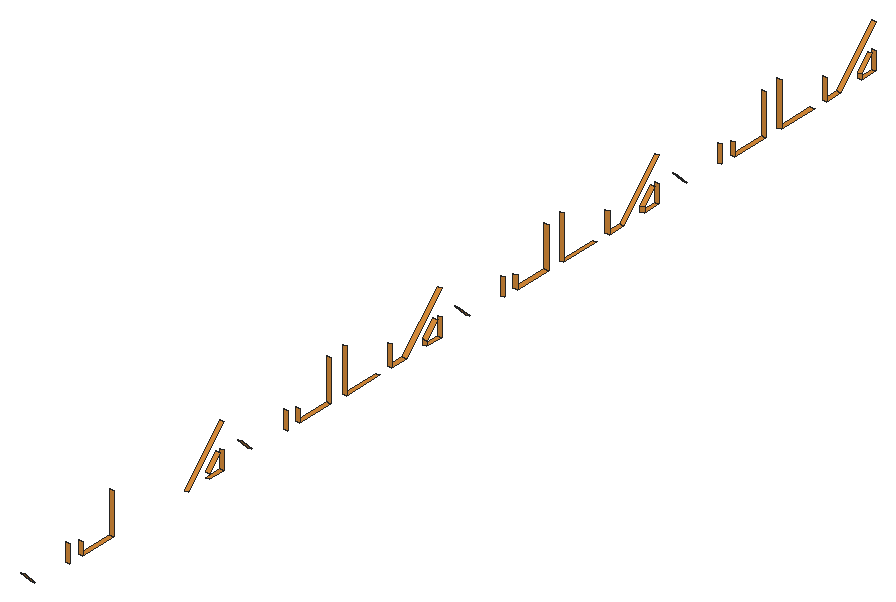
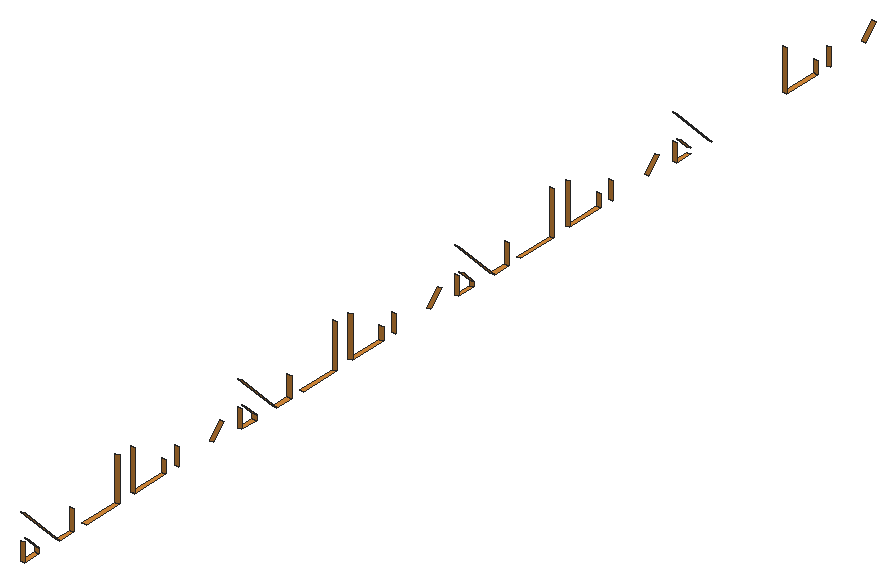
# SketchUp Ruby script. Lengths in inches.
U = 1.inch
M = Sketchup.active_model
def pt(a) = Geom::Point3d.new(a.map { |v| v * U })
def face(e, loops, mat)
  f = e.add_face(loops[0].map { |a| pt(a) })
  loops[1..].each { |l| e.add_face(l.map { |a| pt(a) }).erase! }
  f.material = f.back_material = mat if mat
  f
end
# faces: each face lists its corners as indices into pts; further lists are holes
def faces(e, pts, list, mat = nil) = list.each { |f| face(e, (f[0].is_a?(Array) ? f : [f]).map { |l| l.map { |i| pts[i] } }, mat) }
# xy, xz, yz: faces in a plane at the given z, y or x. An outline is a flat list of corners, or four numbers for a rectangle; further outlines are holes
def ring(l) = l.size == 4 ? [[l[0], l[1]], [l[2], l[1]], [l[2], l[3]], [l[0], l[3]]] : l.each_slice(2).to_a
def flat(e, list, mat, &to3) = list.each { |f| face(e, (f[0].is_a?(Array) ? f : [f]).map { |l| ring(l).map { |u, v| to3.(u, v) } }, mat) }
def xy(e, z, list, mat = nil) = flat(e, list, mat) { |x, y| [x, y, z] }
def xz(e, y, list, mat = nil) = flat(e, list, mat) { |x, z| [x, y, z] }
def yz(e, x, list, mat = nil) = flat(e, list, mat) { |y, z| [x, y, z] }
def lines(e, pts, list) = list.each { |a, b| e.add_line(pt(pts[a]), pt(pts[b])) }
# prism: a flat outline (further loops are holes) pulled along v
def prism(e, loops, v, mat = nil)
  f = face(e, loops, mat); d = Geom::Vector3d.new(v.map { |x| x * U })
  f.pushpull(f.normal.samedirection?(d) ? d.length : -d.length)
end
def box(e, o, s, mat = nil) = prism(e, [[o, [o[0] + s[0], o[1], o[2]], [o[0] + s[0], o[1] + s[1], o[2]], [o[0], o[1] + s[1], o[2]]]], [0, 0, s[2]], mat)
def at(x, y, z, deg = 0) = Geom::Transformation.translation(pt([x, y, z])) * Geom::Transformation.rotation(ORIGIN, Z_AXIS, deg.degrees)
def axes(o, x, y, z) = Geom::Transformation.new([*x, 0, *y, 0, *z, 0, *pt(o).to_a, 1])
def part(name) = M.definitions.add(name)
# library, detail: a bought-in or finely detailed component or shape, given as its bounding box
def library(name, o, s) = part(name).tap { |d| box(d.entities, o, s) }
def detail(e, o, s) = box(e.add_group.entities, o, s)
def put(e, d, t, mat = nil) = e.add_instance(d, t).tap { |i| i.material = mat if mat }
def group(e, t, mat = nil) = e.add_group.tap { |g| g.transformation = t; g.material = mat if mat }.entities
root = M.entities
M.materials.add("1056 AP 9903 Mellow Melon-N").color = [219, 142, 59]
xy(root,148.27,[[14.35,58.41,15.0625,61.42],[14.35,87,15.0625,93.87],[14.35,96.45,15.0625,99.42],[14.35,103.75,15.0625,106.76],[14.35,132.34,15.0625,139.21],
  [14.35,141.79,15.0625,144.77],[14.35,149.1,15.0625,152.1],[14.35,177.68,15.0625,184.56],[14.35,187.14,15.0625,190.11],[14.35,194.44,15.0625,197.45]],"1056 AP 9903 Mellow Melon-N")
xy(root,148.47,[[14.35,31.88,15.0625,38.38],[14.35,77.22,15.0625,83.72],[14.35,122.57,15.0625,129.07],[14.35,167.91,15.0625,174.41]],"1056 AP 9903 Mellow Melon-N")
xz(root,29.28,[[14.35,148.47,15.0625,151.45]],"1056 AP 9903 Mellow Melon-N")
xz(root,31.88,[[14.35,148.47,15.0625,150.62]],"1056 AP 9903 Mellow Melon-N")
xz(root,38.38,[[14.35,148.47,15.0625,155.34]],"1056 AP 9903 Mellow Melon-N")
xz(root,61.42,[[14.35,148.27,15.0625,151.3]],"1056 AP 9903 Mellow Melon-N")
xz(root,74.625,[[14.35,148.47,15.0625,151.45]],"1056 AP 9903 Mellow Melon-N")
xz(root,77.22,[[14.35,148.47,15.0625,150.62]],"1056 AP 9903 Mellow Melon-N")
xz(root,83.72,[[14.35,148.47,15.0625,155.34]],"1056 AP 9903 Mellow Melon-N")
xz(root,87,[[14.35,148.27,15.0625,155.63]],"1056 AP 9903 Mellow Melon-N")
xz(root,96.45,[[14.35,148.27,15.0625,151.76]],"1056 AP 9903 Mellow Melon-N")
xz(root,103.75,[[14.35,148.27,15.0625,149.14]],"1056 AP 9903 Mellow Melon-N")
xz(root,106.76,[[14.35,148.27,15.0625,151.3]],"1056 AP 9903 Mellow Melon-N")
xz(root,119.97,[[14.35,148.47,15.0625,151.45]],"1056 AP 9903 Mellow Melon-N")
xz(root,122.57,[[14.35,148.47,15.0625,150.62]],"1056 AP 9903 Mellow Melon-N")
xz(root,129.07,[[14.35,148.47,15.0625,155.34]],"1056 AP 9903 Mellow Melon-N")
xz(root,132.34,[[14.35,148.27,15.0625,155.63]],"1056 AP 9903 Mellow Melon-N")
xz(root,141.79,[[14.35,148.27,15.0625,151.76]],"1056 AP 9903 Mellow Melon-N")
xz(root,149.1,[[14.35,148.27,15.0625,149.14]],"1056 AP 9903 Mellow Melon-N")
xz(root,152.1,[[14.35,148.27,15.0625,151.3]],"1056 AP 9903 Mellow Melon-N")
xz(root,165.3125,[[14.35,148.47,15.0625,151.45]],"1056 AP 9903 Mellow Melon-N")
xz(root,167.91,[[14.35,148.47,15.0625,150.62]],"1056 AP 9903 Mellow Melon-N")
xz(root,174.41,[[14.35,148.47,15.0625,155.34]],"1056 AP 9903 Mellow Melon-N")
xz(root,177.68,[[14.35,148.27,15.0625,155.63]],"1056 AP 9903 Mellow Melon-N")
xz(root,187.14,[[14.35,148.27,15.0625,151.76]],"1056 AP 9903 Mellow Melon-N")
xz(root,194.44,[[14.35,148.27,15.0625,149.14]],"1056 AP 9903 Mellow Melon-N")
xz(root,197.45,[[14.35,148.27,15.0625,151.3]],"1056 AP 9903 Mellow Melon-N")
p = [[15.0625,54.08,148.27],[15.0625,61.42,155.61],[14.35,61.42,155.61],[14.35,54.08,148.27],[15.0625,99.42,148.27],[15.0625,106.76,155.61],
  [14.35,106.76,155.61],[14.35,99.42,148.27],[15.0625,144.77,148.27],[15.0625,152.11,155.61],[14.35,152.11,155.61],[14.35,144.77,148.27],
  [15.0625,190.11,148.27],[15.0625,197.45,155.61],[14.35,197.45,155.61],[14.35,190.11,148.27],[15.0625,21.91,148.89],[15.0625,19.75,151.05],
  [14.35,19.75,151.05],[14.35,21.91,148.89],[15.0625,67.26,148.89],[15.0625,65.1,151.05],[14.35,65.1,151.05],[14.35,67.26,148.89],
  [15.0625,112.6,148.89],[15.0625,110.44,151.05],[14.35,110.44,151.05],[14.35,112.6,148.89],[15.0625,157.94,148.89],[15.0625,155.79,151.05],
  [14.35,155.79,151.05],[14.35,157.94,148.89],[15.0625,60.57,151.3],[15.0625,58.41,149.14],[14.35,58.41,149.14],[14.35,60.57,151.3],
  [15.0625,105.91,151.3],[15.0625,103.75,149.14],[14.35,103.75,149.14],[14.35,105.91,151.3],[15.0625,151.25,151.3],[15.0625,149.1,149.14],
  [14.35,149.1,149.14],[14.35,151.25,151.3],[15.0625,196.6,151.3],[15.0625,194.44,149.14],[14.35,194.44,149.14],[14.35,196.6,151.3]]
faces(root,p,[[0,1,2,3],[4,5,6,7],[8,9,10,11],[12,13,14,15],[16,17,18,19],[20,21,22,23],[24,25,26,27],[28,29,30,31],
  [32,33,34,35],[36,37,38,39],[40,41,42,43],[44,45,46,47]],"1056 AP 9903 Mellow Melon-N")
